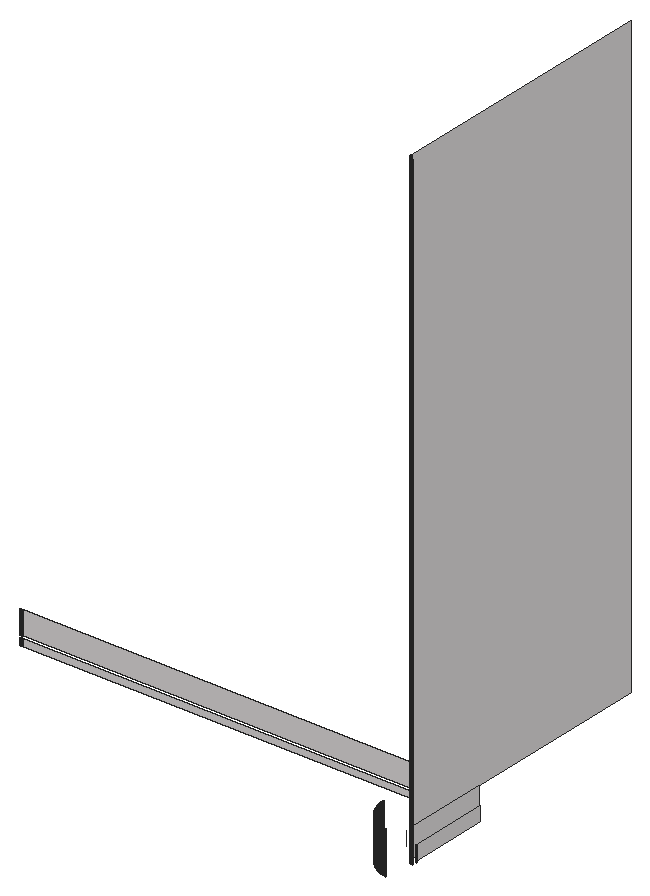
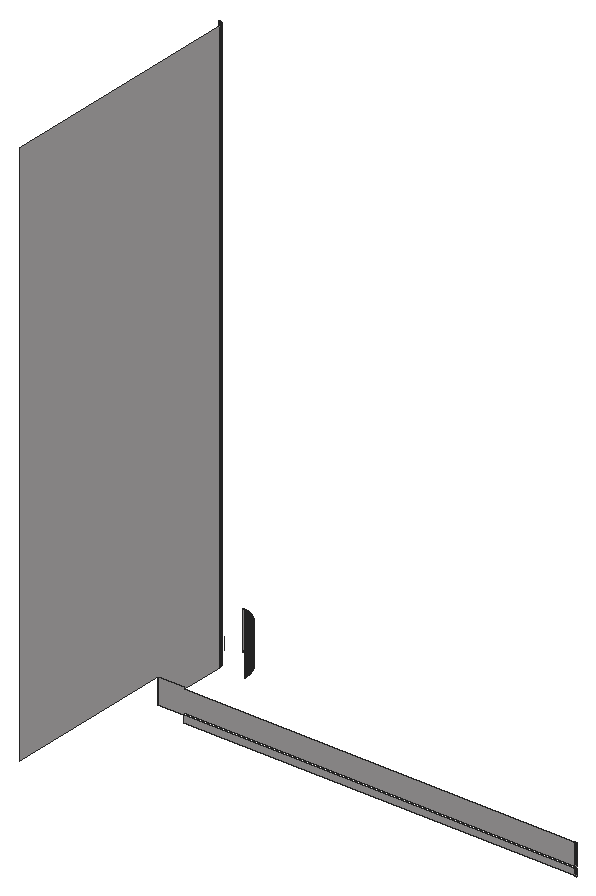
# SketchUp Ruby script. Lengths in inches.
U = 1.inch
M = Sketchup.active_model
def pt(a) = Geom::Point3d.new(a.map { |v| v * U })
def face(e, loops, mat)
  f = e.add_face(loops[0].map { |a| pt(a) })
  loops[1..].each { |l| e.add_face(l.map { |a| pt(a) }).erase! }
  f.material = f.back_material = mat if mat
  f
end
# faces: each face lists its corners as indices into pts; further lists are holes
def faces(e, pts, list, mat = nil) = list.each { |f| face(e, (f[0].is_a?(Array) ? f : [f]).map { |l| l.map { |i| pts[i] } }, mat) }
# xy, xz, yz: faces in a plane at the given z, y or x. An outline is a flat list of corners, or four numbers for a rectangle; further outlines are holes
def ring(l) = l.size == 4 ? [[l[0], l[1]], [l[2], l[1]], [l[2], l[3]], [l[0], l[3]]] : l.each_slice(2).to_a
def flat(e, list, mat, &to3) = list.each { |f| face(e, (f[0].is_a?(Array) ? f : [f]).map { |l| ring(l).map { |u, v| to3.(u, v) } }, mat) }
def xy(e, z, list, mat = nil) = flat(e, list, mat) { |x, y| [x, y, z] }
def xz(e, y, list, mat = nil) = flat(e, list, mat) { |x, z| [x, y, z] }
def yz(e, x, list, mat = nil) = flat(e, list, mat) { |y, z| [x, y, z] }
def lines(e, pts, list) = list.each { |a, b| e.add_line(pt(pts[a]), pt(pts[b])) }
# prism: a flat outline (further loops are holes) pulled along v
def prism(e, loops, v, mat = nil)
  f = face(e, loops, mat); d = Geom::Vector3d.new(v.map { |x| x * U })
  f.pushpull(f.normal.samedirection?(d) ? d.length : -d.length)
end
def box(e, o, s, mat = nil) = prism(e, [[o, [o[0] + s[0], o[1], o[2]], [o[0] + s[0], o[1] + s[1], o[2]], [o[0], o[1] + s[1], o[2]]]], [0, 0, s[2]], mat)
def at(x, y, z, deg = 0) = Geom::Transformation.translation(pt([x, y, z])) * Geom::Transformation.rotation(ORIGIN, Z_AXIS, deg.degrees)
def axes(o, x, y, z) = Geom::Transformation.new([*x, 0, *y, 0, *z, 0, *pt(o).to_a, 1])
def part(name) = M.definitions.add(name)
# library, detail: a bought-in or finely detailed component or shape, given as its bounding box
def library(name, o, s) = part(name).tap { |d| box(d.entities, o, s) }
def detail(e, o, s) = box(e.add_group.entities, o, s)
def put(e, d, t, mat = nil) = e.add_instance(d, t).tap { |i| i.material = mat if mat }
def group(e, t, mat = nil) = e.add_group.tap { |g| g.transformation = t; g.material = mat if mat }.entities
root = M.entities
M.materials.add("[Quartz Light Brown]").color = [215, 212, 212]
xz(root,194,[[18,111,201,114],[201,114,213,114,213,126,201,126,201,125,18,125,18,115,201,115],[201,114,213,126]],"[Quartz Light Brown]")
yz(root,213,[[157.961,114,194,114,194,126,275,126,275,384,157.961,384],[158,114,194,126]],"[Quartz Light Brown]")
yz(root,215,[[158,114,192,120]],"[Quartz Light Brown]")
p = [[16.588,194.055,114],[16.588,194.055,111],[16.823,194.039,111],[16.823,194.039,114],[17.058,194.025,111],[17.058,194.025,114],
  [17.293,194.014,111],[17.293,194.014,114],[17.529,194.006,111],[17.529,194.006,114],[17.764,194.002,111],[17.764,194.002,114],
  [18,194,111],[18,194,114],[213.266,143.251,132],[213.266,143.251,114],[213.46,143.217,114],[213.46,143.217,132],
  [213.653,143.185,114],[213.653,143.185,132],[213.848,143.155,114],[213.848,143.155,132],[212.69,143.37,132],[212.69,143.37,114],
  [212.881,143.328,114],[212.881,143.328,132],[213.074,143.288,114],[213.074,143.288,132],[212.308,143.462,132],[212.308,143.462,114],
  [212.498,143.414,114],[212.498,143.414,132],[211.928,143.563,132],[211.928,143.563,114],[212.118,143.511,114],[212.118,143.511,132],
  [211.552,143.675,132],[211.552,143.675,114],[211.74,143.618,114],[211.74,143.618,132],[211.178,143.796,132],[211.178,143.796,114],
  [211.365,143.734,114],[211.365,143.734,132],[210.993,143.86,132],[210.993,143.86,114],[210.624,143.996,132],[210.624,143.996,114],
  [210.808,143.927,114],[210.808,143.927,132],[210.442,144.068,132],[210.442,144.068,114],[210.079,144.218,132],[210.079,144.218,114],
  [210.26,144.142,114],[210.26,144.142,132],[209.899,144.297,132],[209.899,144.297,114],[209.72,144.378,132],[209.72,144.378,114],
  [209.542,144.461,132],[209.542,144.461,114],[209.19,144.635,132],[209.19,144.635,114],[209.366,144.547,114],[209.366,144.547,132],
  [209.016,144.725,132],[209.016,144.725,114],[208.843,144.818,132],[208.843,144.818,114],[208.671,144.913,132],[208.671,144.913,114],
  [208.5,145.01,132],[208.5,145.01,114],[208.331,145.109,132],[208.331,145.109,114],[208.163,145.21,132],[208.163,145.21,114],
  [207.996,145.314,132],[207.996,145.314,114],[207.83,145.42,132],[207.83,145.42,114],[207.666,145.528,132],[207.666,145.528,114],
  [207.504,145.638,132],[207.504,145.638,114],[207.343,145.75,132],[207.343,145.75,114],[207.183,145.865,132],[207.183,145.865,114],
  [207.025,145.981,132],[207.025,145.981,114],[206.869,146.1,132],[206.869,146.1,114],[206.714,146.22,132],[206.714,146.22,114],
  [206.56,146.343,132],[206.56,146.343,114],[206.408,146.467,132],[206.408,146.467,114],[206.258,146.594,132],[206.258,146.594,114],
  [206.11,146.722,132],[206.11,146.722,114],[205.963,146.853,132],[205.963,146.853,114],[205.818,146.985,132],[205.818,146.985,114],
  [205.675,147.119,132],[205.675,147.119,114],[205.533,147.255,132],[205.533,147.255,114],[205.393,147.393,132],[205.393,147.393,114],
  [205.255,147.533,132],[205.255,147.533,114],[205.119,147.675,132],[205.119,147.675,114],[204.985,147.818,132],[204.985,147.818,114],
  [204.853,147.963,132],[204.853,147.963,114],[204.722,148.11,132],[204.722,148.11,114],[204.594,148.258,132],[204.594,148.258,114],
  [204.467,148.408,132],[204.467,148.408,114],[204.343,148.56,132],[204.343,148.56,114],[204.22,148.714,132],[204.22,148.714,114],
  [204.1,148.869,132],[204.1,148.869,114],[203.981,149.025,132],[203.981,149.025,114],[203.865,149.183,132],[203.865,149.183,114],
  [203.75,149.343,132],[203.75,149.343,114],[203.638,149.504,132],[203.638,149.504,114],[203.528,149.666,132],[203.528,149.666,114],
  [203.42,149.83,132],[203.42,149.83,114],[203.314,149.996,132],[203.314,149.996,114],[203.21,150.163,132],[203.21,150.163,114],
  [203.109,150.331,132],[203.109,150.331,114],[203.01,150.5,132],[203.01,150.5,114],[202.913,150.671,132],[202.913,150.671,114],
  [202.818,150.843,132],[202.818,150.843,114],[202.725,151.016,132],[202.725,151.016,114],[202.635,151.19,132],[202.635,151.19,114],
  [202.547,151.366,132],[202.547,151.366,114],[202.461,151.542,132],[202.461,151.542,114],[202.378,151.72,132],[202.378,151.72,114],
  [202.297,151.899,132],[202.297,151.899,114],[202.218,152.079,132],[202.218,152.079,114],[202.142,152.26,132],[202.142,152.26,114],
  [202.068,152.442,132],[202.068,152.442,114],[201.996,152.624,132],[201.996,152.624,114],[201.927,152.808,132],[201.927,152.808,114],
  [201.86,152.993,132],[201.86,152.993,114],[201.796,153.178,132],[201.796,153.178,114],[201.734,153.365,132],[201.734,153.365,114],
  [201.675,153.552,132],[201.675,153.552,114],[201.618,153.74,132],[201.618,153.74,114],[201.563,153.928,132],[201.563,153.928,114],
  [201.511,154.118,132],[201.511,154.118,114],[201.462,154.308,132],[201.462,154.308,114],[201.414,154.498,132],[201.414,154.498,114],
  [201.37,154.69,132],[201.37,154.69,114],[201.328,154.881,132],[201.328,154.881,114],[201.288,155.074,132],[201.288,155.074,114],
  [215.531,155.037,126],[215.415,155.058,126],[215.415,155.058,114],[215.531,155.037,114],[215.528,155.037,114],[215.412,155.058,114],
  [215.412,155.058,126],[215.412,155.058,384],[215.415,155.058,384],[215.453,155.05,384],[215.492,155.043,384],[215.528,155.037,384],
  [215.528,155.037,126],[215.648,155.021,126],[215.648,155.021,114],[215.644,155.021,114],[215.531,155.037,384],[215.57,155.031,384],
  [215.608,155.026,384],[215.644,155.021,384],[215.644,155.021,126],[215.765,155.009,126],[215.765,155.009,114],[215.761,155.01,114],
  [215.647,155.021,384],[215.686,155.016,384],[215.725,155.013,384],[215.761,155.01,384],[215.761,155.01,126],[215.882,155.002,126],
  [215.882,155.002,114],[215.879,155.002,114],[215.765,155.009,384],[215.804,155.006,384],[215.843,155.004,384],[215.879,155.002,384],
  [215.879,155.002,126],[215.921,155.001,114],[215.88,155.002,384],[215.882,155.002,384],[215.921,155.001,384],[215.921,155.001,126],
  [215.961,155,384],[215.961,155,114],[201.251,155.266,132],[201.251,155.266,114],[215.073,155.147,126],[214.962,155.185,126],
  [214.962,155.185,114],[215.073,155.147,114],[215.07,155.148,114],[214.959,155.186,114],[214.959,155.186,126],[214.959,155.186,384],
  [214.962,155.185,384],[214.999,155.172,384],[215.036,155.159,384],[215.07,155.148,384],[215.07,155.148,126],[215.186,155.113,126],
  [215.186,155.113,114],[215.183,155.113,114],[215.073,155.147,384],[215.11,155.135,384],[215.148,155.124,384],[215.183,155.113,384],
  [215.183,155.113,126],[215.3,155.083,126],[215.3,155.083,114],[215.297,155.084,114],[215.186,155.113,384],[215.224,155.102,384],
  [215.262,155.092,384],[215.297,155.084,384],[215.297,155.084,126],[215.3,155.083,384],[215.338,155.074,384],[215.376,155.066,384],
  [214.852,155.228,126],[214.744,155.276,126],[214.744,155.276,114],[214.852,155.228,114],[214.85,155.229,114],[214.742,155.277,114],
  [214.742,155.277,126],[214.742,155.277,384],[214.744,155.276,384],[214.78,155.259,384],[214.816,155.244,384],[214.85,155.229,384],
  [214.85,155.229,126],[214.852,155.228,384],[214.888,155.214,384],[214.925,155.199,384],[201.217,155.46,132],[201.217,155.46,114],
  [214.638,155.327,126],[214.534,155.383,126],[214.534,155.383,114],[214.638,155.327,114],[214.636,155.328,114],[214.532,155.384,114],
  [214.532,155.384,126],[214.532,155.384,384],[214.534,155.383,384],[214.569,155.364,384],[214.603,155.345,384],[214.636,155.328,384],
  [214.636,155.328,126],[214.638,155.327,384],[214.673,155.309,384],[214.708,155.292,384],[214.433,155.442,126],[214.333,155.506,126],
  [214.333,155.506,114],[214.433,155.442,114],[214.431,155.443,114],[214.332,155.507,114],[214.332,155.507,126],[214.332,155.507,384],
  [214.333,155.506,384],[214.366,155.484,384],[214.399,155.463,384],[214.431,155.443,384],[214.431,155.443,126],[214.433,155.442,384],
  [214.466,155.422,384],[214.5,155.402,384],[201.185,155.653,132],[201.185,155.653,114],[214.237,155.573,126],[214.237,155.573,114],
  [214.235,155.574,114],[214.235,155.574,126],[214.235,155.574,384],[214.237,155.573,384],[214.269,155.55,384],[214.301,155.528,384],
  [214.143,155.644,126],[214.052,155.719,126],[214.052,155.719,114],[214.143,155.644,114],[214.142,155.645,114],[214.051,155.72,114],
  [214.051,155.72,126],[214.051,155.72,384],[214.052,155.719,384],[214.082,155.693,384],[214.112,155.669,384],[214.142,155.645,384],
  [214.141,155.645,126],[214.143,155.644,384],[214.174,155.62,384],[214.205,155.596,384],[201.155,155.848,132],[201.155,155.848,114],
  [213.964,155.797,126],[213.964,155.797,114],[213.963,155.798,114],[213.963,155.798,126],[213.963,155.798,384],[213.964,155.797,384],
  [213.993,155.771,384],[214.022,155.744,384],[201.128,156.042,132],[201.128,156.042,114],[213.879,155.879,126],[213.879,155.879,114],
  [213.878,155.88,114],[213.878,155.88,126],[213.878,155.88,384],[213.879,155.879,384],[213.907,155.851,384],[213.935,155.824,384],
  [213.797,155.964,126],[213.797,155.964,114],[213.796,155.965,114],[213.796,155.964,126],[213.796,155.965,384],[213.797,155.964,384],
  [213.824,155.935,384],[213.851,155.907,384],[201.104,156.237,132],[201.104,156.237,114],[213.719,156.052,126],[213.719,156.052,114],
  [213.718,156.052,114],[213.719,156.052,126],[213.719,156.052,384],[213.744,156.022,384],[213.771,155.993,384],[213.644,156.143,126],
  [213.573,156.237,126],[213.573,156.237,114],[213.644,156.143,114],[213.644,156.143,114],[213.573,156.237,114],[213.573,156.237,126],
  [213.573,156.237,384],[213.596,156.205,384],[213.62,156.174,384],[213.644,156.143,384],[213.644,156.143,126],[213.669,156.112,384],
  [213.693,156.082,384],[201.082,156.432,132],[201.082,156.432,114],[213.506,156.333,126],[213.506,156.333,114],[213.505,156.334,114],
  [213.506,156.333,126],[213.506,156.333,384],[213.528,156.301,384],[213.55,156.269,384],[213.442,156.433,126],[213.442,156.433,114],
  [213.442,156.433,114],[213.442,156.433,126],[213.442,156.433,384],[213.463,156.399,384],[213.484,156.366,384],[201.063,156.627,132],
  [201.063,156.627,114],[213.383,156.534,126],[213.383,156.534,114],[213.382,156.535,114],[213.383,156.534,126],[213.383,156.534,384],
  [213.402,156.5,384],[213.422,156.466,384],[213.327,156.638,126],[213.327,156.638,114],[213.327,156.638,114],[213.327,156.638,126],
  [213.327,156.638,384],[213.345,156.603,384],[213.364,156.569,384],[201.046,156.823,132],[201.046,156.823,114],[213.276,156.744,126],
  [213.276,156.744,114],[213.276,156.744,114],[213.276,156.744,126],[213.276,156.744,384],[213.292,156.708,384],[213.309,156.673,384],
  [213.229,156.852,126],[213.229,156.852,114],[213.229,156.852,114],[213.228,156.852,126],[213.228,156.852,384],[213.244,156.816,384],
  [213.259,156.78,384],[201.032,157.019,132],[201.032,157.019,114],[213.186,156.962,126],[213.186,156.962,114],[213.186,156.962,114],
  [213.185,156.962,126],[213.185,156.962,384],[213.199,156.925,384],[213.214,156.888,384],[201.021,157.215,132],[201.021,157.215,114],
  [213.147,157.073,126],[213.147,157.073,114],[213.147,157.073,114],[213.147,157.073,126],[213.147,157.073,384],[213.159,157.036,384],
  [213.159,157.036,126],[213.172,156.999,126],[213.172,156.999,384],[215.691,157.049,114],[215.654,157.062,114],[215.654,157.062,120],
  [215.691,157.049,120],[215.729,157.038,114],[215.729,157.038,120],[215.767,157.028,114],[215.767,157.028,120],[215.805,157.019,114],
  [215.805,157.019,120],[215.844,157.012,114],[215.844,157.012,120],[215.883,157.007,114],[215.883,157.007,120],[215.922,157.003,114],
  [215.922,157.003,120],[213.113,157.186,126],[213.113,157.186,114],[213.113,157.185,114],[213.113,157.186,126],[213.113,157.186,384],
  [213.124,157.148,384],[213.124,157.148,126],[213.135,157.11,126],[213.135,157.11,384],[215.478,157.147,114],[215.445,157.169,114],
  [215.445,157.169,120],[215.478,157.147,120],[215.512,157.128,114],[215.512,157.128,120],[215.546,157.109,114],[215.546,157.109,120],
  [215.582,157.092,114],[215.582,157.092,120],[215.617,157.076,114],[215.617,157.076,120],[201.012,157.411,132],[201.012,157.411,114],
  [213.083,157.3,126],[213.083,157.3,114],[213.083,157.299,114],[213.083,157.3,126],[213.083,157.3,384],[213.092,157.262,384],
  [213.102,157.224,384],[215.351,157.24,114],[215.321,157.266,114],[215.321,157.266,120],[215.351,157.24,120],[215.381,157.215,114],
  [215.381,157.215,120],[215.412,157.191,114],[215.412,157.191,120],[213.058,157.415,126],[213.058,157.415,114],[213.058,157.414,114],
  [213.058,157.415,126],[213.058,157.415,384],[213.066,157.376,384],[213.074,157.338,384],[215.266,157.321,114],[215.24,157.351,114],
  [215.24,157.351,120],[215.266,157.321,120],[215.293,157.293,114],[215.293,157.293,120],[201.005,157.607,132],[201.005,157.607,114],
  [213.037,157.531,126],[213.037,157.531,114],[213.037,157.53,114],[213.037,157.531,126],[213.037,157.531,384],[213.043,157.492,384],
  [213.05,157.453,384],[215.169,157.444,114],[215.148,157.478,114],[215.148,157.478,120],[215.169,157.444,120],[215.191,157.412,114],
  [215.191,157.412,120],[215.215,157.381,114],[215.215,157.381,120],[213.021,157.647,126],[213.021,157.647,114],[213.021,157.647,114],
  [213.021,157.647,126],[213.021,157.647,384],[213.026,157.608,384],[213.031,157.57,384],[215.109,157.546,114],[215.092,157.581,114],
  [215.092,157.581,120],[215.109,157.546,120],[215.128,157.511,114],[215.128,157.511,120],[201.001,157.804,132],[201.001,157.804,114],
  [213.009,157.765,126],[213.009,157.765,114],[213.01,157.764,114],[213.009,157.765,126],[213.009,157.765,384],[213.013,157.725,384],
  [213.016,157.686,384],[215.076,157.617,114],[215.062,157.654,114],[215.062,157.654,120],[215.076,157.617,120],[215.038,157.729,114],
  [215.028,157.767,114],[215.028,157.767,120],[215.038,157.729,120],[215.049,157.691,114],[215.049,157.691,120],[201,158,132],
  [201,158,114],[213.002,157.882,126],[213.002,157.882,114],[213.003,157.881,114],[213.002,157.881,126],[213.003,157.881,384],
  [213.004,157.843,384],[213.006,157.804,384],[215.012,157.844,114],[215.007,157.882,114],[215.007,157.882,120],[215.012,157.844,120],
  [215.019,157.805,114],[215.019,157.805,120],[213,158,126],[213,158,114],[213,157.961,384],[213.001,157.921,384],
  [213.001,157.921,126],[213.001,157.921,114],[213,157.961,114],[213.002,157.882,384],[215.003,157.922,114],[215.001,157.961,114],
  [215.001,157.961,120],[215.003,157.922,120],[215,158,114],[215,158,120],[16.588,194.055,125],[16.588,194.055,115],
  [16.823,194.039,115],[16.823,194.039,125],[17.058,194.025,115],[17.058,194.025,125],[17.293,194.014,115],[17.293,194.014,125],
  [17.529,194.006,115],[17.529,194.006,125],[17.764,194.002,115],[17.764,194.002,125],[18,194,115],[18,194,125],
  [213,155,120],[213,155,126]]
faces(root,p,[[0,1,2,3],[3,2,4,5],[5,4,6,7],[7,6,8,9],[9,8,10,11],[11,10,12,13],[14,15,16,17],[17,16,18,19],
  [19,18,20,21],[22,23,24,25],[25,24,26,27],[27,26,15,14],[28,29,30,31],[31,30,23,22],[32,33,34,35],[35,34,29,28],
  [36,37,38,39],[39,38,33,32],[40,41,42,43],[43,42,37,36],[44,45,41,40],[46,47,48,49],[49,48,45,44],[50,51,47,46],
  [52,53,54,55],[55,54,51,50],[56,57,53,52],[58,59,57,56],[60,61,59,58],[62,63,64,65],[65,64,61,60],[66,67,63,62],
  [68,69,67,66],[70,71,69,68],[72,73,71,70],[74,75,73,72],[76,77,75,74],[78,79,77,76],[80,81,79,78],[82,83,81,80],
  [84,85,83,82],[86,87,85,84],[88,89,87,86],[90,91,89,88],[92,93,91,90],[94,95,93,92],[96,97,95,94],[98,99,97,96],
  [100,101,99,98],[102,103,101,100],[104,105,103,102],[106,107,105,104],[108,109,107,106],[110,111,109,108],[112,113,111,110],[114,115,113,112],
  [116,117,115,114],[118,119,117,116],[120,121,119,118],[122,123,121,120],[124,125,123,122],[126,127,125,124],[128,129,127,126],[130,131,129,128],
  [132,133,131,130],[134,135,133,132],[136,137,135,134],[138,139,137,136],[140,141,139,138],[142,143,141,140],[144,145,143,142],[146,147,145,144],
  [148,149,147,146],[150,151,149,148],[152,153,151,150],[154,155,153,152],[156,157,155,154],[158,159,157,156],[160,161,159,158],[162,163,161,160],
  [164,165,163,162],[166,167,165,164],[168,169,167,166],[170,171,169,168],[172,173,171,170],[174,175,173,172],[176,177,175,174],[178,179,177,176],
  [180,181,179,178],[182,183,181,180],[184,185,183,182],[186,187,185,184],[188,189,187,186],[190,191,189,188],[192,193,191,190],[194,195,193,192],
  [196,197,195,194],[198,199,197,196],[200,201,199,198],[202,203,201,200],[204,205,206,207],[208,209,210,211,212,213,214,215,216],[217,204,207,218],[219,208,216,215,220,221,222,223,224],
  [225,217,218,226],[227,219,224,223,228,229,230,231,232],[233,225,226,234],[235,227,232,231,236,237,238,239,240],[241,235,240,239,242,243,244,245],[245,244,246,247,241],[248,249,203,202],[250,251,252,253],
  [254,255,256,257,258,259,260,261,262],[263,250,253,264],[265,254,262,261,266,267,268,269,270],[271,263,264,272],[273,265,270,269,274,275,276,277,278],[205,271,272,206],[209,273,278,277,279,280,281,211,210],[282,283,284,285],
  [286,287,288,289,290,291,292,293,294],[255,286,294,293,295,296,297,257,256],[251,282,285,252],[298,299,249,248],[300,301,302,303],[304,305,306,307,308,309,310,311,312],[283,300,303,284],[287,304,312,311,313,314,315,289,288],
  [316,317,318,319],[320,321,322,323,324,325,326,327,328],[301,316,319,302],[305,320,328,327,329,330,331,307,306],[332,333,299,298],[317,334,335,318],[321,336,337,338,339,340,341,323,322],[342,343,344,345],
  [334,342,345,335],[346,347,348,349,350,351,352,353,354],[336,346,354,353,355,356,357,338,337],[358,359,333,332],[343,360,361,344],[347,362,363,364,365,366,367,349,348],[368,369,359,358],[360,370,371,361],
  [362,372,373,374,375,376,377,364,363],[370,378,379,371],[372,380,381,382,383,384,385,374,373],[386,387,369,368],[378,388,389,379],[380,390,391,392,393,394,382,381],[395,396,397,398],[388,395,398,389],
  [399,400,401,402,403,404,405,406],[390,399,406,405,407,408,392,391],[409,410,387,386],[396,411,412,397],[400,413,414,415,416,417,402,401],[411,418,419,412],[413,420,421,422,423,424,415,414],[425,426,410,409],
  [418,427,428,419],[420,429,430,431,432,433,422,421],[427,434,435,428],[429,436,437,438,439,440,431,430],[441,442,426,425],[434,443,444,435],[436,445,446,447,448,449,438,437],[443,450,451,444],
  [445,452,453,454,455,456,447,446],[457,458,442,441],[450,459,460,451],[452,461,462,463,464,465,454,453],[466,467,458,457],[459,468,469,460],[461,470,471,472,473,474,475,476,463,462],[477,478,479,480],
  [481,477,480,482],[483,481,482,484],[485,483,484,486],[487,485,486,488],[489,487,488,490],[491,489,490,492],[468,493,494,469],[470,495,496,497,498,499,500,501,472,471],
  [502,503,504,505],[506,502,505,507],[508,506,507,509],[510,508,509,511],[512,510,511,513],[478,512,513,479],[514,515,467,466],[493,516,517,494],
  [495,518,519,520,521,522,497,496],[523,524,525,526],[527,523,526,528],[529,527,528,530],[503,529,530,504],[516,531,532,517],[518,533,534,535,536,537,520,519],[538,539,540,541],
  [542,538,541,543],[524,542,543,525],[544,545,515,514],[531,546,547,532],[533,548,549,550,551,552,535,534],[553,554,555,556],[557,553,556,558],[559,557,558,560],
  [539,559,560,540],[546,561,562,547],[548,563,564,565,566,567,550,549],[568,569,570,571],[572,568,571,573],[554,572,573,555],[574,575,545,544],[561,576,577,562],
  [563,578,579,580,581,582,565,564],[583,584,585,586],[569,583,586,570],[587,588,589,590],[591,587,590,592],[584,591,592,585],[593,594,575,574],[576,595,596,577],
  [578,597,598,599,600,601,580,579],[602,603,604,605],[606,602,605,607],[588,606,607,589],[595,608,609,596],[610,611,612,613,614],[597,613,612,611,615,599,598],[616,617,618,619],
  [603,616,619,604],[617,620,621,618],[622,623,624,625],[625,624,626,627],[627,626,628,629],[629,628,630,631],[631,630,632,633],[633,632,634,635]],"[Quartz Light Brown]")
lines(root,p,[[636,637]])
